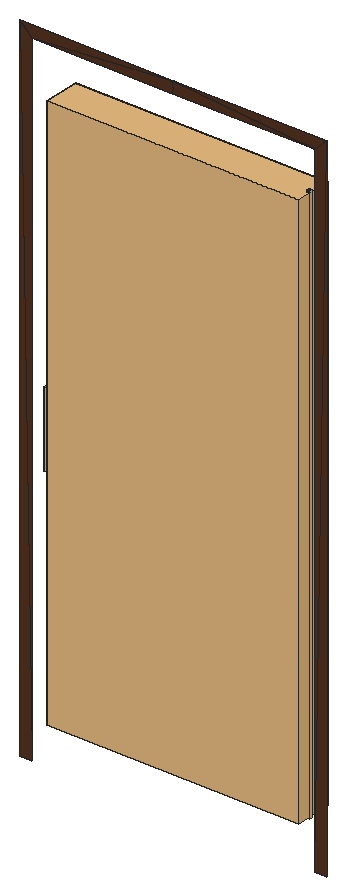
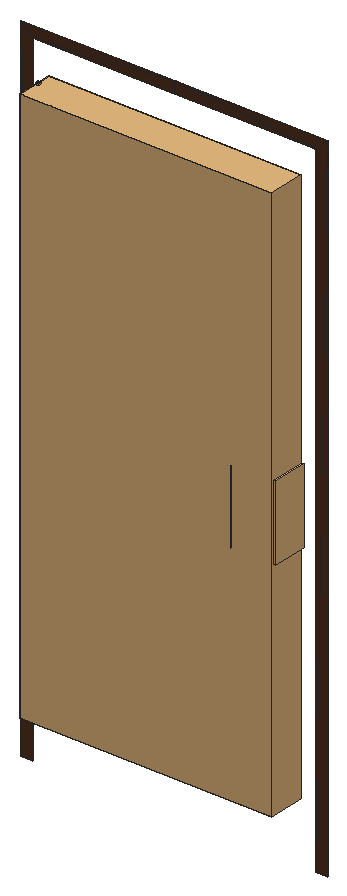
# SketchUp Ruby script. Lengths in inches.
U = 1.inch
M = Sketchup.active_model
def pt(a) = Geom::Point3d.new(a.map { |v| v * U })
def face(e, loops, mat)
  f = e.add_face(loops[0].map { |a| pt(a) })
  loops[1..].each { |l| e.add_face(l.map { |a| pt(a) }).erase! }
  f.material = f.back_material = mat if mat
  f
end
# faces: each face lists its corners as indices into pts; further lists are holes
def faces(e, pts, list, mat = nil) = list.each { |f| face(e, (f[0].is_a?(Array) ? f : [f]).map { |l| l.map { |i| pts[i] } }, mat) }
# xy, xz, yz: faces in a plane at the given z, y or x. An outline is a flat list of corners, or four numbers for a rectangle; further outlines are holes
def ring(l) = l.size == 4 ? [[l[0], l[1]], [l[2], l[1]], [l[2], l[3]], [l[0], l[3]]] : l.each_slice(2).to_a
def flat(e, list, mat, &to3) = list.each { |f| face(e, (f[0].is_a?(Array) ? f : [f]).map { |l| ring(l).map { |u, v| to3.(u, v) } }, mat) }
def xy(e, z, list, mat = nil) = flat(e, list, mat) { |x, y| [x, y, z] }
def xz(e, y, list, mat = nil) = flat(e, list, mat) { |x, z| [x, y, z] }
def yz(e, x, list, mat = nil) = flat(e, list, mat) { |y, z| [x, y, z] }
def lines(e, pts, list) = list.each { |a, b| e.add_line(pt(pts[a]), pt(pts[b])) }
# prism: a flat outline (further loops are holes) pulled along v
def prism(e, loops, v, mat = nil)
  f = face(e, loops, mat); d = Geom::Vector3d.new(v.map { |x| x * U })
  f.pushpull(f.normal.samedirection?(d) ? d.length : -d.length)
end
def box(e, o, s, mat = nil) = prism(e, [[o, [o[0] + s[0], o[1], o[2]], [o[0] + s[0], o[1] + s[1], o[2]], [o[0], o[1] + s[1], o[2]]]], [0, 0, s[2]], mat)
def at(x, y, z, deg = 0) = Geom::Transformation.translation(pt([x, y, z])) * Geom::Transformation.rotation(ORIGIN, Z_AXIS, deg.degrees)
def axes(o, x, y, z) = Geom::Transformation.new([*x, 0, *y, 0, *z, 0, *pt(o).to_a, 1])
def part(name) = M.definitions.add(name)
# library, detail: a bought-in or finely detailed component or shape, given as its bounding box
def library(name, o, s) = part(name).tap { |d| box(d.entities, o, s) }
def detail(e, o, s) = box(e.add_group.entities, o, s)
def put(e, d, t, mat = nil) = e.add_instance(d, t).tap { |i| i.material = mat if mat }
def group(e, t, mat = nil) = e.add_group.tap { |g| g.transformation = t; g.material = mat if mat }.entities
root = M.entities
M.materials.add("Material \#0").color = [86, 53, 35]
M.materials.add("Material \#1").color = [140, 140, 140]
c1 = library("3DGeom~9_Defintion",[456.52,-471.89,-18.89],[5.57,1000,5.49])
c2 = library("3DGeom~7_Defintion",[455.56,-471.94,-18.85],[5.55,1000,5.48])
c3 = part("3DGeom~8_Defintion")
xz(c3.entities,-471.94,[[458.125,-17.29,459.53,-16.11,457.73,-17.15],[458.125,-17.29,458.54,-17.29,459.53,-16.11],[458.54,-17.29,458.93,-17.15,459.53,-16.11],[457.73,-17.15,459.53,-16.11,457.42,-16.88],[458.93,-17.15,459.25,-16.88,459.53,-16.11],
  [457.42,-16.88,459.53,-16.11,457.21,-16.52],[459.25,-16.88,459.46,-16.52,459.53,-16.11],[457.21,-16.52,459.53,-16.11,457.14,-16.11],[457.14,-16.11,459.53,-16.11,457.21,-15.7],[459.53,-16.11,457.42,-15.34,457.21,-15.7],
  [459.53,-16.11,457.73,-15.07,457.42,-15.34],[459.53,-16.11,458.125,-14.93,457.73,-15.07],[459.53,-16.11,458.54,-14.93,458.125,-14.93],[459.53,-16.11,458.93,-15.07,458.54,-14.93],[459.53,-16.11,459.25,-15.34,458.93,-15.07],
  [459.53,-16.11,459.46,-15.7,459.25,-15.34]],"Material \#1")
xz(c3.entities,-416.39,[[458.125,-17.29,457.73,-17.15,459.53,-16.11],[458.125,-17.29,459.53,-16.11,458.54,-17.29],[458.54,-17.29,459.53,-16.11,458.93,-17.15],[457.73,-17.15,457.42,-16.88,459.53,-16.11],[458.93,-17.15,459.53,-16.11,459.25,-16.88],
  [457.42,-16.88,457.21,-16.52,459.53,-16.11],[459.25,-16.88,459.53,-16.11,459.46,-16.52],[457.21,-16.52,457.14,-16.11,459.53,-16.11],[457.14,-16.11,457.21,-15.7,459.53,-16.11],[459.53,-16.11,457.21,-15.7,457.42,-15.34],
  [459.53,-16.11,457.42,-15.34,457.73,-15.07],[459.53,-16.11,457.73,-15.07,458.125,-14.93],[459.53,-16.11,458.125,-14.93,458.54,-14.93],[459.53,-16.11,458.54,-14.93,458.93,-15.07],[459.53,-16.11,458.93,-15.07,459.25,-15.34],
  [459.53,-16.11,459.25,-15.34,459.46,-15.7]],"Material \#1")
xz(c3.entities,-27.5,[[458.125,-17.29,459.53,-16.11,457.73,-17.15],[458.125,-17.29,458.54,-17.29,459.53,-16.11],[458.54,-17.29,458.93,-17.15,459.53,-16.11],[457.73,-17.15,459.53,-16.11,457.42,-16.88],[458.93,-17.15,459.25,-16.88,459.53,-16.11],
  [457.42,-16.88,459.53,-16.11,457.21,-16.52],[459.25,-16.88,459.46,-16.52,459.53,-16.11],[457.21,-16.52,459.53,-16.11,457.14,-16.11],[457.14,-16.11,459.53,-16.11,457.21,-15.7],[459.53,-16.11,457.42,-15.34,457.21,-15.7],
  [459.53,-16.11,457.73,-15.07,457.42,-15.34],[459.53,-16.11,458.125,-14.93,457.73,-15.07],[459.53,-16.11,458.54,-14.93,458.125,-14.93],[459.53,-16.11,458.93,-15.07,458.54,-14.93],[459.53,-16.11,459.25,-15.34,458.93,-15.07],
  [459.53,-16.11,459.46,-15.7,459.25,-15.34]],"Material \#1")
xz(c3.entities,28.06,[[458.125,-17.29,457.73,-17.15,459.53,-16.11],[458.125,-17.29,459.53,-16.11,458.54,-17.29],[458.54,-17.29,459.53,-16.11,458.93,-17.15],[457.73,-17.15,457.42,-16.88,459.53,-16.11],[458.93,-17.15,459.53,-16.11,459.25,-16.88],
  [457.42,-16.88,457.21,-16.52,459.53,-16.11],[459.25,-16.88,459.53,-16.11,459.46,-16.52],[457.21,-16.52,457.14,-16.11,459.53,-16.11],[457.14,-16.11,457.21,-15.7,459.53,-16.11],[459.53,-16.11,457.21,-15.7,457.42,-15.34],
  [459.53,-16.11,457.42,-15.34,457.73,-15.07],[459.53,-16.11,457.73,-15.07,458.125,-14.93],[459.53,-16.11,458.125,-14.93,458.54,-14.93],[459.53,-16.11,458.54,-14.93,458.93,-15.07],[459.53,-16.11,458.93,-15.07,459.25,-15.34],
  [459.53,-16.11,459.25,-15.34,459.46,-15.7]],"Material \#1")
xz(c3.entities,472.5,[[458.125,-17.29,459.53,-16.11,457.73,-17.15],[458.125,-17.29,458.54,-17.29,459.53,-16.11],[458.54,-17.29,458.93,-17.15,459.53,-16.11],[457.73,-17.15,459.53,-16.11,457.42,-16.88],[458.93,-17.15,459.25,-16.88,459.53,-16.11],
  [457.42,-16.88,459.53,-16.11,457.21,-16.52],[459.25,-16.88,459.46,-16.52,459.53,-16.11],[457.21,-16.52,459.53,-16.11,457.14,-16.11],[457.14,-16.11,459.53,-16.11,457.21,-15.7],[459.53,-16.11,457.42,-15.34,457.21,-15.7],
  [459.53,-16.11,457.73,-15.07,457.42,-15.34],[459.53,-16.11,458.125,-14.93,457.73,-15.07],[459.53,-16.11,458.54,-14.93,458.125,-14.93],[459.53,-16.11,458.93,-15.07,458.54,-14.93],[459.53,-16.11,459.25,-15.34,458.93,-15.07],
  [459.53,-16.11,459.46,-15.7,459.25,-15.34]],"Material \#1")
xz(c3.entities,528.06,[[458.125,-17.29,457.73,-17.15,459.53,-16.11],[458.125,-17.29,459.53,-16.11,458.54,-17.29],[458.54,-17.29,459.53,-16.11,458.93,-17.15],[457.73,-17.15,457.42,-16.88,459.53,-16.11],[458.93,-17.15,459.53,-16.11,459.25,-16.88],
  [457.42,-16.88,457.21,-16.52,459.53,-16.11],[459.25,-16.88,459.53,-16.11,459.46,-16.52],[457.21,-16.52,457.14,-16.11,459.53,-16.11],[457.14,-16.11,457.21,-15.7,459.53,-16.11],[459.53,-16.11,457.21,-15.7,457.42,-15.34],
  [459.53,-16.11,457.42,-15.34,457.73,-15.07],[459.53,-16.11,457.73,-15.07,458.125,-14.93],[459.53,-16.11,458.125,-14.93,458.54,-14.93],[459.53,-16.11,458.54,-14.93,458.93,-15.07],[459.53,-16.11,458.93,-15.07,459.25,-15.34],
  [459.53,-16.11,459.25,-15.34,459.46,-15.7]],"Material \#1")
c4 = part("3DGeom~21_Defintion")
xy(c4.entities,73.08,[[-976.3,-241.71,23.7,-241.71,-976.3,-223.46],[23.7,-241.71,5.45,-223.46,-976.3,-223.46],[23.7,-241.71,23.7,0,5.45,-223.46],[5.45,-223.46,23.7,0,5.45,0],[23.7,0,23.7,241.71,5.45,223.46],
  [5.45,0,23.7,0,5.45,223.46],[-976.3,223.46,23.7,241.71,-976.3,241.71],[-976.3,223.46,5.45,223.46,23.7,241.71]],"Material \#0")
c5 = library("3DGeom~6_Defintion",[-5.59,-471.8,-48.03],[468.87,1000,73.72])
c6 = library("3DGeom~3_Defintion",[-83.33,-500,-350],[620.1,1000,533.33])
xy(root,-3.87,[[371.22,117.13,371.16,117.15,371.17,117.17],[371.22,117.13,371.17,117.17,371.23,117.15],[371.22,117.13,371.23,117.15,371.29,117.13],[371.29,117.13,371.23,117.15,371.29,117.15],[371.29,117.13,371.29,117.15,371.36,117.15],
  [371.16,117.15,371.1,117.19,371.12,117.2],[371.16,117.15,371.12,117.2,371.17,117.17],[371.29,117.15,371.35,117.17,371.36,117.15],[371.36,117.15,371.35,117.17,371.42,117.19],[371.35,117.17,371.4,117.2,371.42,117.19],
  [371.1,117.19,371.07,117.25,371.08,117.25],[371.1,117.19,371.08,117.25,371.12,117.2],[371.42,117.19,371.4,117.2,371.45,117.25],[371.4,117.2,371.43,117.25,371.45,117.25],[371.07,117.25,371.05,117.3125,371.07,117.3125],
  [371.07,117.25,371.07,117.3125,371.08,117.25],[371.43,117.25,371.44,117.3125,371.47,117.3125],[371.43,117.25,371.47,117.3125,371.45,117.25],[371.05,117.3125,371.07,117.375,371.08,117.37],[371.05,117.3125,371.08,117.37,371.07,117.3125],
  [371.44,117.3125,371.43,117.37,371.45,117.375],[371.44,117.3125,371.45,117.375,371.47,117.3125],[371.08,117.37,371.07,117.375,371.12,117.42],[371.43,117.37,371.4,117.42,371.42,117.43],[371.43,117.37,371.42,117.43,371.45,117.375],
  [371.07,117.375,371.1,117.43,371.12,117.42],[371.12,117.42,371.1,117.43,371.17,117.46],[371.4,117.42,371.35,117.46,371.36,117.47],[371.4,117.42,371.36,117.47,371.42,117.43],[371.1,117.43,371.16,117.47,371.17,117.46],
  [371.17,117.46,371.16,117.47,371.23,117.48],[371.35,117.46,371.29,117.48,371.29,117.5],[371.35,117.46,371.29,117.5,371.36,117.47],[371.16,117.47,371.22,117.5,371.23,117.48],[371.23,117.48,371.22,117.5,371.29,117.48],
  [371.29,117.48,371.22,117.5,371.29,117.5]],"Material \#1")
xy(root,-3.85,[[371.22,117.13,371.23,117.15,371.16,117.15],[371.22,117.13,371.29,117.13,371.29,117.15],[371.22,117.13,371.29,117.15,371.23,117.15],[371.29,117.13,371.35,117.17,371.29,117.15],[371.29,117.13,371.36,117.15,371.35,117.17],
  [371.16,117.15,371.17,117.17,371.1,117.19],[371.16,117.15,371.23,117.15,371.17,117.17],[371.36,117.15,371.4,117.2,371.35,117.17],[371.36,117.15,371.42,117.19,371.4,117.2],[371.17,117.17,371.12,117.2,371.1,117.19],
  [371.1,117.19,371.12,117.2,371.07,117.25],[371.42,117.19,371.43,117.25,371.4,117.2],[371.42,117.19,371.45,117.25,371.43,117.25],[371.12,117.2,371.08,117.25,371.07,117.25],[371.07,117.25,371.08,117.25,371.05,117.3125],
  [371.08,117.25,371.07,117.3125,371.05,117.3125],[371.43,117.25,371.45,117.25,371.44,117.3125],[371.45,117.25,371.47,117.3125,371.44,117.3125],[371.05,117.3125,371.07,117.3125,371.07,117.375],[371.07,117.3125,371.08,117.37,371.07,117.375],
  [371.44,117.3125,371.47,117.3125,371.43,117.37],[371.47,117.3125,371.45,117.375,371.43,117.37],[371.08,117.37,371.1,117.43,371.07,117.375],[371.08,117.37,371.12,117.42,371.1,117.43],[371.43,117.37,371.45,117.375,371.4,117.42],
  [371.45,117.375,371.42,117.43,371.4,117.42],[371.12,117.42,371.16,117.47,371.1,117.43],[371.12,117.42,371.17,117.46,371.16,117.47],[371.4,117.42,371.42,117.43,371.35,117.46],[371.42,117.43,371.36,117.47,371.35,117.46],
  [371.17,117.46,371.22,117.5,371.16,117.47],[371.17,117.46,371.23,117.48,371.22,117.5],[371.35,117.46,371.36,117.47,371.29,117.48],[371.36,117.47,371.29,117.5,371.29,117.48],[371.23,117.48,371.29,117.5,371.22,117.5],
  [371.23,117.48,371.29,117.48,371.29,117.5]],"Material \#1")
xy(root,0,[[371.22,117.13,371.16,117.15,371.23,117.15],[371.22,117.13,371.23,117.15,371.29,117.15],[371.22,117.13,371.29,117.15,371.29,117.13],[371.29,117.13,371.29,117.15,371.35,117.17],[371.29,117.13,371.35,117.17,371.36,117.15],
  [371.16,117.15,371.1,117.19,371.17,117.17],[371.16,117.15,371.17,117.17,371.23,117.15],[371.36,117.15,371.35,117.17,371.4,117.2],[371.36,117.15,371.4,117.2,371.42,117.19],[371.17,117.17,371.1,117.19,371.12,117.2],
  [371.1,117.19,371.07,117.25,371.12,117.2],[371.42,117.19,371.4,117.2,371.43,117.25],[371.42,117.19,371.43,117.25,371.45,117.25],[371.12,117.2,371.07,117.25,371.08,117.25],[371.07,117.25,371.05,117.3125,371.08,117.25],
  [371.08,117.25,371.05,117.3125,371.07,117.3125],[371.43,117.25,371.44,117.3125,371.45,117.25],[371.45,117.25,371.44,117.3125,371.47,117.3125],[371.05,117.3125,371.07,117.375,371.07,117.3125],[371.07,117.3125,371.07,117.375,371.08,117.37],
  [371.44,117.3125,371.43,117.37,371.47,117.3125],[371.47,117.3125,371.43,117.37,371.45,117.375],[371.08,117.37,371.07,117.375,371.1,117.43],[371.08,117.37,371.1,117.43,371.12,117.42],[371.43,117.37,371.4,117.42,371.45,117.375],
  [371.45,117.375,371.4,117.42,371.42,117.43],[371.12,117.42,371.1,117.43,371.16,117.47],[371.12,117.42,371.16,117.47,371.17,117.46],[371.4,117.42,371.35,117.46,371.42,117.43],[371.42,117.43,371.35,117.46,371.36,117.47],
  [371.17,117.46,371.16,117.47,371.22,117.5],[371.17,117.46,371.22,117.5,371.23,117.48],[371.35,117.46,371.29,117.48,371.36,117.47],[371.36,117.47,371.29,117.48,371.29,117.5],[371.23,117.48,371.22,117.5,371.29,117.5],
  [371.23,117.48,371.29,117.5,371.29,117.48]],"Material \#1")
xy(root,0.02,[[371.22,117.13,371.17,117.17,371.16,117.15],[371.22,117.13,371.23,117.15,371.17,117.17],[371.22,117.13,371.29,117.13,371.23,117.15],[371.29,117.13,371.29,117.15,371.23,117.15],[371.29,117.13,371.36,117.15,371.29,117.15],
  [371.16,117.15,371.12,117.2,371.1,117.19],[371.16,117.15,371.17,117.17,371.12,117.2],[371.29,117.15,371.36,117.15,371.35,117.17],[371.36,117.15,371.42,117.19,371.35,117.17],[371.35,117.17,371.42,117.19,371.4,117.2],
  [371.1,117.19,371.08,117.25,371.07,117.25],[371.1,117.19,371.12,117.2,371.08,117.25],[371.42,117.19,371.45,117.25,371.4,117.2],[371.4,117.2,371.45,117.25,371.43,117.25],[371.07,117.25,371.07,117.3125,371.05,117.3125],
  [371.07,117.25,371.08,117.25,371.07,117.3125],[371.43,117.25,371.45,117.25,371.47,117.3125],[371.43,117.25,371.47,117.3125,371.44,117.3125],[371.05,117.3125,371.07,117.3125,371.08,117.37],[371.05,117.3125,371.08,117.37,371.07,117.375],
  [371.44,117.3125,371.45,117.375,371.43,117.37],[371.44,117.3125,371.47,117.3125,371.45,117.375],[371.08,117.37,371.12,117.42,371.07,117.375],[371.43,117.37,371.42,117.43,371.4,117.42],[371.43,117.37,371.45,117.375,371.42,117.43],
  [371.07,117.375,371.12,117.42,371.1,117.43],[371.12,117.42,371.17,117.46,371.1,117.43],[371.4,117.42,371.36,117.47,371.35,117.46],[371.4,117.42,371.42,117.43,371.36,117.47],[371.1,117.43,371.17,117.46,371.16,117.47],
  [371.17,117.46,371.23,117.48,371.16,117.47],[371.35,117.46,371.29,117.5,371.29,117.48],[371.35,117.46,371.36,117.47,371.29,117.5],[371.16,117.47,371.23,117.48,371.22,117.5],[371.23,117.48,371.29,117.48,371.22,117.5],
  [371.29,117.48,371.29,117.5,371.22,117.5]],"Material \#1")
xz(root,116.5625,[[337.22,27.35,337.22,27.37,337.35,27.38],[337.22,27.35,337.35,27.38,337.35,27.37],[337.35,27.37,337.35,27.38,337.47,27.41],[337.35,27.37,337.47,27.41,337.47,27.4],[337.47,27.4,337.47,27.41,337.58,27.47],
  [337.47,27.4,337.58,27.47,337.58,27.46],[337.58,27.46,337.58,27.47,337.68,27.54],[337.58,27.46,337.68,27.54,337.68,27.53],[337.68,27.53,337.68,27.54,337.76,27.63],[337.68,27.53,337.76,27.63,337.77,27.62],
  [337.22,27.56,337.22,27.57,337.26,27.57],[337.22,27.56,337.26,27.57,337.26,27.56],[337.26,27.56,337.26,27.57,337.3,27.58],[337.26,27.56,337.3,27.58,337.3,27.57],[337.3,27.57,337.3,27.58,337.33,27.6],
  [337.3,27.57,337.33,27.6,337.34,27.59],[337.34,27.59,337.33,27.6,337.37,27.625],[337.34,27.59,337.37,27.625,337.375,27.61],[337.375,27.61,337.37,27.625,337.39,27.65],[337.375,27.61,337.39,27.65,337.4,27.64],
  [337.77,27.62,337.76,27.63,337.83,27.73],[337.77,27.62,337.83,27.73,337.84,27.73],[337.4,27.64,337.39,27.65,337.41,27.69],[337.4,27.64,337.41,27.69,337.43,27.68],[337.43,27.68,337.41,27.69,337.43,27.72],
  [337.83,27.73,337.88,27.85,337.84,27.73],[337.84,27.73,337.88,27.85,337.9,27.84],[337.9,27.84,337.88,27.85,337.92,27.97],[337.9,27.84,337.92,27.97,337.93,27.97],[337.92,27.97,337.93,28.11,337.93,27.97],
  [337.93,27.97,337.93,28.11,337.94,28.11],[337.33,28.01,337.3,28.03,337.34,28.02],[337.34,28.02,337.3,28.03,337.3,28.04],[337.3,28.03,337.26,28.04,337.3,28.04],[337.22,28.04,337.22,28.05,337.26,28.05],
  [337.22,28.04,337.26,28.05,337.26,28.04],[337.26,28.04,337.26,28.05,337.3,28.04],[337.93,28.11,337.93,34.84,337.94,28.11]],"Material \#1")
xz(root,118.74,[[337.77,27.62,337.83,27.73,337.76,27.63],[337.77,27.62,337.84,27.73,337.83,27.73],[337.43,27.68,337.44,27.72,337.43,27.72],[337.43,27.72,337.44,27.72,337.44,27.76],[337.83,27.73,337.84,27.73,337.88,27.85],
  [337.84,27.73,337.9,27.84,337.88,27.85],[337.46,27.8,337.45,27.85,337.44,27.85],[337.9,27.84,337.92,27.97,337.88,27.85],[337.9,27.84,337.93,27.97,337.92,27.97],[337.45,27.85,337.44,27.89,337.43,27.89],
  [337.92,27.97,337.93,27.97,337.93,28.11],[337.93,27.97,337.94,28.11,337.93,28.11],[337.93,28.11,337.94,28.11,337.93,34.84],[337.94,28.11,337.93,36.6875,337.93,34.84],[337.94,28.11,337.94,36.6875,337.93,36.6875]],"Material \#1")
p = [[337.15,118.74,27.76],[337.14,118.74,27.73],[337.14,118.71,27.73],[337.15,118.71,27.76],[337.12,118.73,27.71],[337.12,118.7,27.71],
  [337.14,118.73,27.6875],[337.14,118.7,27.6875],[337.16,118.73,27.67],[337.16,118.7,27.67],[337.18,118.74,27.7],[337.18,118.71,27.7],
  [337.2,118.74,27.72],[337.2,118.71,27.72],[337.29,118.74,27.85],[337.29,118.71,27.85],[337.24,118.74,27.89],[337.24,118.71,27.89],
  [337.26,118.74,27.91],[337.26,118.71,27.91],[337.3,118.74,27.88],[337.3,118.71,27.88],[337.32,118.73,27.9],[337.32,118.7,27.9],
  [337.3,118.73,27.92],[337.3,118.7,27.92],[337.27,118.73,27.9375],[337.27,118.7,27.9375]]
faces(root,p,[[0,1,2],[2,3,0],[1,4,5],[5,2,1],[4,6,7],[7,5,4],[6,8,9],[9,7,6],
  [8,10,11],[11,9,8],[10,12,13],[13,11,10],[12,14,15],[15,13,12],[16,0,3],[3,17,16],
  [18,16,17],[17,19,18],[14,20,21],[21,15,14],[20,22,23],[23,21,20],[22,24,25],[25,23,22],
  [24,26,27],[27,25,24],[26,18,19],[19,27,26]],"Material \#1")
put(root,c1,axes([337.22,118.4,32.4],[0.07411,0,0],[0,0,0.07711],[0,0.06738,0]),"Material \#1")
put(root,c2,axes([337.22,118.4,32.4],[0.07427,0,0],[0,0,0.07728],[0,0.06752,0]),"Material \#1")
put(root,c3,axes([337.22,118.4,32.4],[0.07427,0,0],[0,0,0.07728],[0,0.06752,0]),"Material \#1")
put(root,c4,axes([352.49,123.125,77.91],[0,0,0.09059],[0.08706,0,0],[0,-0.07915,0]),"Material \#0")
put(root,c5,axes([337.22,118.4,32.4],[0.07388,0,0],[0,0,0.07687],[0,0.06716,0]),"Material \#1")
put(root,c6,axes([337.22,118.4,32.4],[0.0099,0,0],[0,0,0.0103],[0,0.009,0]),"Material \#1")
